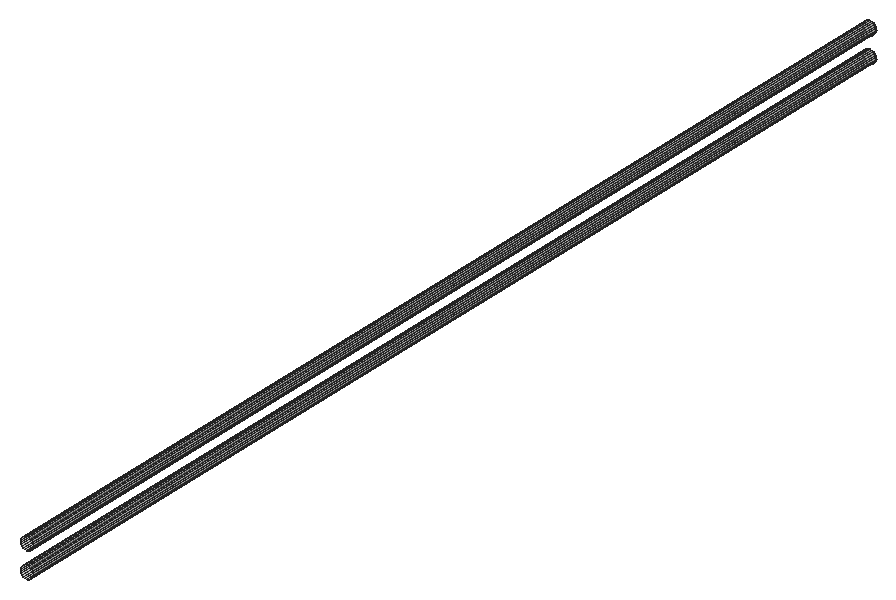
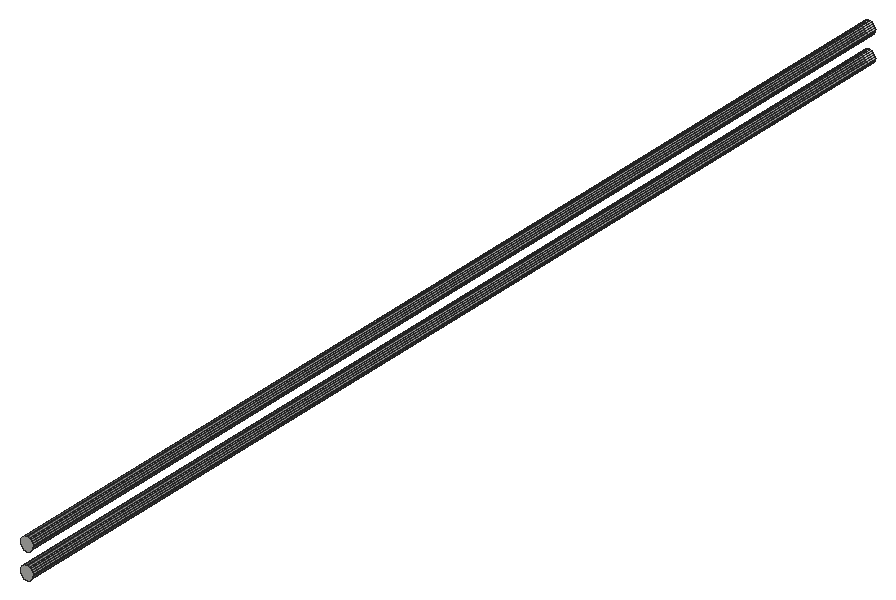
# SketchUp Ruby script. Lengths in inches.
U = 1.inch
M = Sketchup.active_model
def pt(a) = Geom::Point3d.new(a.map { |v| v * U })
def face(e, loops, mat)
  f = e.add_face(loops[0].map { |a| pt(a) })
  loops[1..].each { |l| e.add_face(l.map { |a| pt(a) }).erase! }
  f.material = f.back_material = mat if mat
  f
end
# faces: each face lists its corners as indices into pts; further lists are holes
def faces(e, pts, list, mat = nil) = list.each { |f| face(e, (f[0].is_a?(Array) ? f : [f]).map { |l| l.map { |i| pts[i] } }, mat) }
# xy, xz, yz: faces in a plane at the given z, y or x. An outline is a flat list of corners, or four numbers for a rectangle; further outlines are holes
def ring(l) = l.size == 4 ? [[l[0], l[1]], [l[2], l[1]], [l[2], l[3]], [l[0], l[3]]] : l.each_slice(2).to_a
def flat(e, list, mat, &to3) = list.each { |f| face(e, (f[0].is_a?(Array) ? f : [f]).map { |l| ring(l).map { |u, v| to3.(u, v) } }, mat) }
def xy(e, z, list, mat = nil) = flat(e, list, mat) { |x, y| [x, y, z] }
def xz(e, y, list, mat = nil) = flat(e, list, mat) { |x, z| [x, y, z] }
def yz(e, x, list, mat = nil) = flat(e, list, mat) { |y, z| [x, y, z] }
def lines(e, pts, list) = list.each { |a, b| e.add_line(pt(pts[a]), pt(pts[b])) }
# prism: a flat outline (further loops are holes) pulled along v
def prism(e, loops, v, mat = nil)
  f = face(e, loops, mat); d = Geom::Vector3d.new(v.map { |x| x * U })
  f.pushpull(f.normal.samedirection?(d) ? d.length : -d.length)
end
def box(e, o, s, mat = nil) = prism(e, [[o, [o[0] + s[0], o[1], o[2]], [o[0] + s[0], o[1] + s[1], o[2]], [o[0], o[1] + s[1], o[2]]]], [0, 0, s[2]], mat)
def at(x, y, z, deg = 0) = Geom::Transformation.translation(pt([x, y, z])) * Geom::Transformation.rotation(ORIGIN, Z_AXIS, deg.degrees)
def axes(o, x, y, z) = Geom::Transformation.new([*x, 0, *y, 0, *z, 0, *pt(o).to_a, 1])
def part(name) = M.definitions.add(name)
# library, detail: a bought-in or finely detailed component or shape, given as its bounding box
def library(name, o, s) = part(name).tap { |d| box(d.entities, o, s) }
def detail(e, o, s) = box(e.add_group.entities, o, s)
def put(e, d, t, mat = nil) = e.add_instance(d, t).tap { |i| i.material = mat if mat }
def group(e, t, mat = nil) = e.add_group.tap { |g| g.transformation = t; g.material = mat if mat }.entities
root = M.entities
M.materials.add("[Aluminum]").color = [150, 150, 150]
M.materials["[Aluminum]"].alpha = 0.5
xy(root,129.71,[[869.01,117.53,869.09,278.08]],"[Aluminum]")
xy(root,131.7,[[869.09,117.53,869.17,278.08]],"[Aluminum]")
xy(root,133.65,[[869.01,117.53,869.09,278.08]],"[Aluminum]")
xy(root,135.64,[[869.09,117.53,869.17,278.08]],"[Aluminum]")
xz(root,278.08,[[869.01,129.71,868.75,129.76,868.52,129.88,868.33,130.06,868.19,130.28,868.11,130.53,868.09,130.79,868.15,131.04,868.27,131.27,868.44,131.47,868.66,131.61,868.91,131.6875,869.09,131.7,869.17,131.7,869.43,131.65,869.66,131.53,869.85,131.35,869.99,131.13,870.07,130.88,870.09,130.62,870.03,130.37,869.91,130.14,869.74,129.94,869.52,129.8,869.27,129.72,869.09,129.71],[869.01,133.65,868.75,133.7,868.52,133.82,868.33,134,868.19,134.22,868.11,134.47,868.09,134.73,868.15,134.98,868.27,135.21,868.44,135.41,868.66,135.55,868.91,135.63,869.09,135.64,869.17,135.64,869.43,135.59,869.66,135.47,869.85,135.29,869.99,135.07,870.07,134.82,870.09,134.5625,870.03,134.31,869.91,134.08,869.74,133.88,869.52,133.74,869.27,133.66,869.09,133.65]])
p = [[869.01,117.53,129.71],[868.75,117.53,129.76],[868.75,278.08,129.76],[869.01,278.08,129.71],[869.27,117.53,129.72],[869.09,117.53,129.71],
  [869.09,278.08,129.71],[869.27,278.08,129.72],[869.52,117.53,129.8],[869.52,278.08,129.8],[868.52,117.53,129.88],[868.52,278.08,129.88],
  [869.74,117.53,129.94],[869.74,278.08,129.94],[868.33,117.53,130.06],[868.33,278.08,130.06],[869.91,117.53,130.14],[869.91,278.08,130.14],
  [868.19,117.53,130.28],[868.19,278.08,130.28],[870.03,117.53,130.37],[870.03,278.08,130.37],[868.11,117.53,130.53],[868.11,278.08,130.53],
  [870.09,117.53,130.62],[870.09,278.08,130.62],[868.09,117.53,130.79],[868.09,278.08,130.79],[870.07,117.53,130.88],[870.07,278.08,130.88],
  [868.15,117.53,131.04],[868.15,278.08,131.04],[869.99,117.53,131.13],[869.99,278.08,131.13],[868.27,117.53,131.27],[868.27,278.08,131.27],
  [869.85,117.53,131.35],[869.85,278.08,131.35],[868.44,117.53,131.47],[868.44,278.08,131.47],[869.66,117.53,131.53],[869.66,278.08,131.53],
  [868.66,117.53,131.61],[868.66,278.08,131.61],[869.43,117.53,131.65],[869.43,278.08,131.65],[868.91,117.53,131.6875],[868.91,278.08,131.6875],
  [869.17,117.53,131.7],[869.17,278.08,131.7],[869.09,117.53,131.7],[869.09,278.08,131.7],[869.01,117.53,133.65],[868.75,117.53,133.7],
  [868.75,278.08,133.7],[869.01,278.08,133.65],[868.52,117.53,133.82],[868.52,278.08,133.82],[869.27,117.53,133.66],[869.09,117.53,133.65],
  [869.09,278.08,133.65],[869.27,278.08,133.66],[869.52,117.53,133.74],[869.52,278.08,133.74],[869.74,117.53,133.88],[869.74,278.08,133.88],
  [868.33,117.53,134],[868.33,278.08,134],[869.91,117.53,134.08],[869.91,278.08,134.08],[868.19,117.53,134.22],[868.19,278.08,134.22],
  [870.03,117.53,134.31],[870.03,278.08,134.31],[868.11,117.53,134.47],[868.11,278.08,134.47],[870.09,117.53,134.5625],[870.09,278.08,134.5625],
  [868.09,117.53,134.73],[868.09,278.08,134.73],[870.07,117.53,134.82],[870.07,278.08,134.82],[868.15,117.53,134.98],[868.15,278.08,134.98],
  [869.99,117.53,135.07],[869.99,278.08,135.07],[868.27,117.53,135.21],[868.27,278.08,135.21],[869.85,117.53,135.29],[869.85,278.08,135.29],
  [868.44,117.53,135.41],[868.44,278.08,135.41],[869.66,117.53,135.47],[869.66,278.08,135.47],[868.66,117.53,135.55],[868.66,278.08,135.55],
  [868.91,117.53,135.63],[868.91,278.08,135.63],[869.43,117.53,135.59],[869.43,278.08,135.59],[869.09,117.53,135.64],[869.09,278.08,135.64],
  [869.17,117.53,135.64],[869.17,278.08,135.64]]
faces(root,p,[[0,1,2,3],[4,5,6,7],[8,4,7,9],[1,10,11,2],[12,8,9,13],[10,14,15,11],[16,12,13,17],[14,18,19,15],
  [20,16,17,21],[18,22,23,19],[24,20,21,25],[22,26,27,23],[28,24,25,29],[26,30,31,27],[32,28,29,33],[30,34,35,31],
  [36,32,33,37],[34,38,39,35],[40,36,37,41],[38,42,43,39],[44,40,41,45],[42,46,47,43],[48,44,45,49],[46,50,51,47],
  [52,53,54,55],[53,56,57,54],[58,59,60,61],[62,58,61,63],[64,62,63,65],[56,66,67,57],[68,64,65,69],[66,70,71,67],
  [72,68,69,73],[70,74,75,71],[76,72,73,77],[74,78,79,75],[80,76,77,81],[78,82,83,79],[84,80,81,85],[82,86,87,83],
  [88,84,85,89],[86,90,91,87],[92,88,89,93],[90,94,95,91],[94,96,97,95],[98,92,93,99],[96,100,101,97],[102,98,99,103]],"[Aluminum]")
